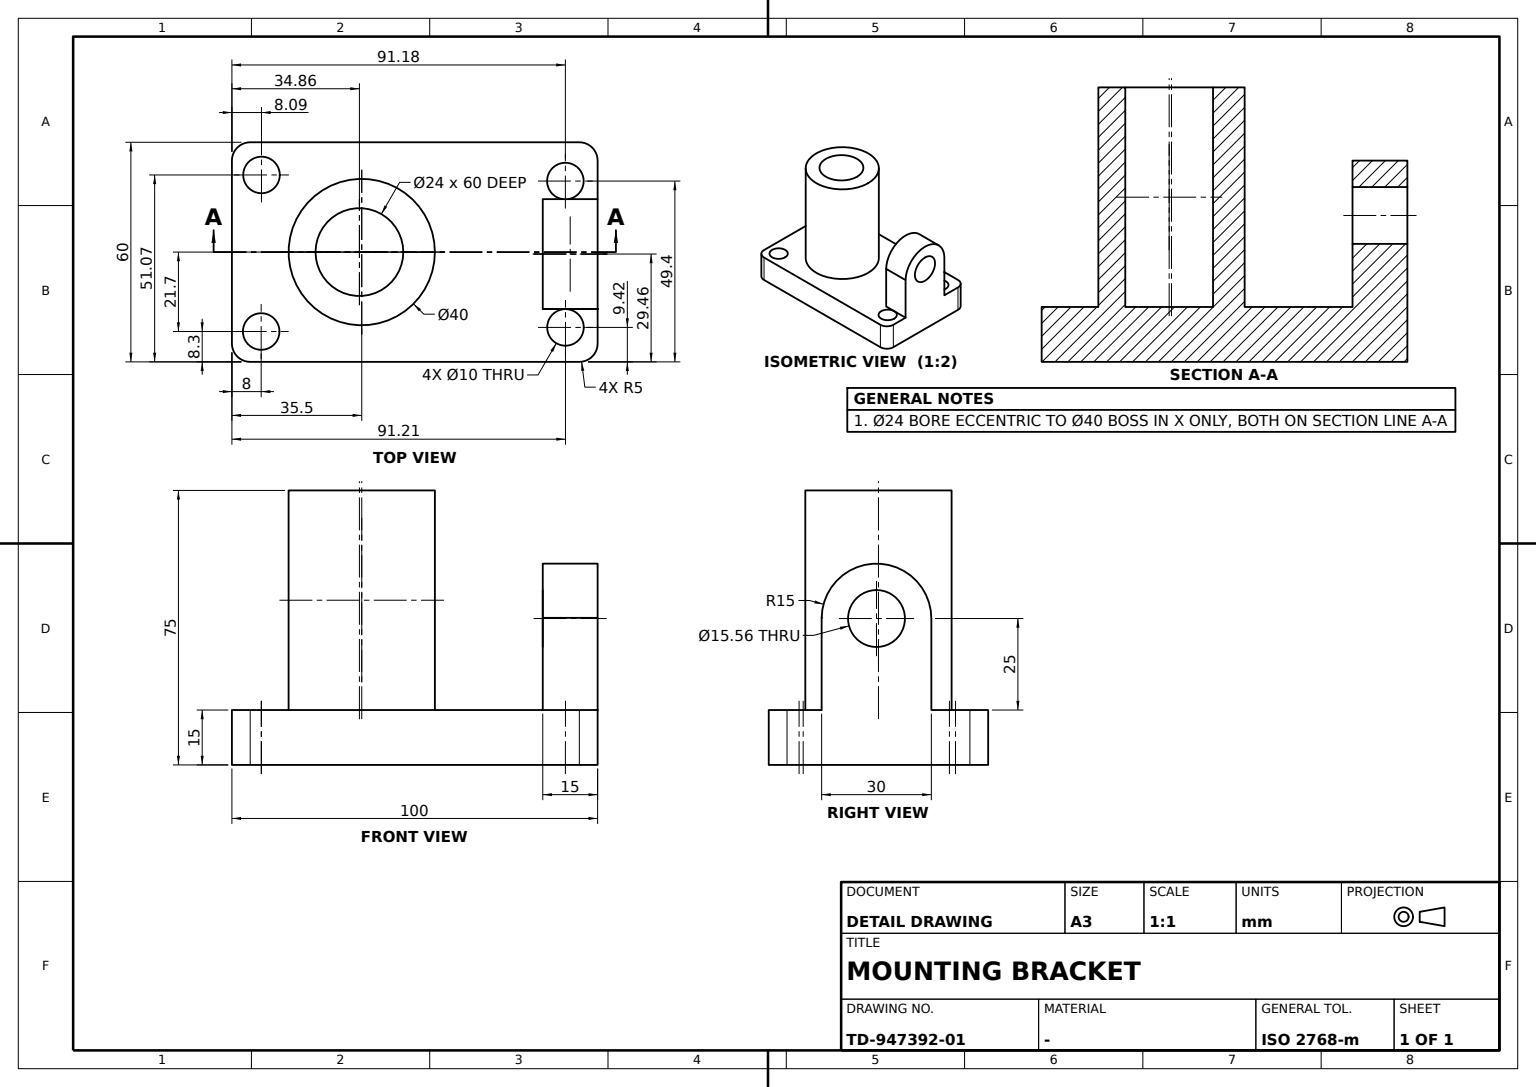
ISO-10303-21;
HEADER;
FILE_DESCRIPTION((''),'2;1');
FILE_NAME('','',(''),(''),'','','');
FILE_SCHEMA(('AUTOMOTIVE_DESIGN'));
ENDSEC;
DATA;
#1=APPLICATION_CONTEXT('');
#2=PRODUCT_CONTEXT('',#1,'mechanical');
#3=PRODUCT('','','',(#2));
#4=PRODUCT_DEFINITION_FORMATION('','',#3);
#5=PRODUCT_DEFINITION_CONTEXT('',#1,'design');
#6=PRODUCT_DEFINITION('','',#4,#5);
#7=PRODUCT_DEFINITION_SHAPE('','',#6);
#8=(LENGTH_UNIT()NAMED_UNIT(*)SI_UNIT(.MILLI.,.METRE.));
#9=(NAMED_UNIT(*)PLANE_ANGLE_UNIT()SI_UNIT($,.RADIAN.));
#10=(NAMED_UNIT(*)SI_UNIT($,.STERADIAN.)SOLID_ANGLE_UNIT());
#11=UNCERTAINTY_MEASURE_WITH_UNIT(LENGTH_MEASURE(0.005),#8,'distance_accuracy_value','');
#12=(GEOMETRIC_REPRESENTATION_CONTEXT(3)GLOBAL_UNCERTAINTY_ASSIGNED_CONTEXT((#11))GLOBAL_UNIT_ASSIGNED_CONTEXT((#8,#9,#10))REPRESENTATION_CONTEXT('',''));
#13=CARTESIAN_POINT('',(58.479646,14.464148,15.));
#14=VERTEX_POINT('',#13);
#15=CARTESIAN_POINT('',(60.042129,14.464148,15.));
#16=VERTEX_POINT('',#15);
#17=CARTESIAN_POINT('',(59.260888,19.402737,15.));
#18=DIRECTION('',(0.,0.,1.));
#19=DIRECTION('',(1.,0.,0.));
#20=AXIS2_PLACEMENT_3D('',#17,#18,#19);
#21=CIRCLE('',#20,5.);
#22=EDGE_CURVE('',#14,#16,#21,.T.);
#23=ORIENTED_EDGE('',*,*,#22,.F.);
#24=CARTESIAN_POINT('',(68.078188,14.464148,15.));
#25=DIRECTION('',(-1.,0.,0.));
#26=VECTOR('',#25,1000.);
#27=LINE('',#24,#26);
#28=EDGE_CURVE('',#16,#14,#27,.T.);
#29=ORIENTED_EDGE('',*,*,#28,.F.);
#30=EDGE_LOOP('',(#23,#29));
#31=FACE_BOUND('',#30,.T.);
#32=CARTESIAN_POINT('',(0.,0.,15.));
#33=AXIS2_PLACEMENT_3D('',#32,#18,#19);
#34=PLANE('',#33);
#35=ADVANCED_FACE('',(#31),#34,.F.);
#36=CARTESIAN_POINT('',(14.941721,0.,75.));
#37=VERTEX_POINT('',#36);
#38=CARTESIAN_POINT('',(2.941721,0.,75.));
#39=AXIS2_PLACEMENT_3D('',#38,#18,#19);
#40=CIRCLE('',#39,12.);
#41=EDGE_CURVE('',#37,#37,#40,.T.);
#42=ORIENTED_EDGE('',*,*,#41,.F.);
#43=EDGE_LOOP('',(#42));
#44=FACE_BOUND('',#43,.T.);
#45=CARTESIAN_POINT('',(23.581214,0.,75.));
#46=VERTEX_POINT('',#45);
#47=CARTESIAN_POINT('',(3.581214,0.,75.));
#48=AXIS2_PLACEMENT_3D('',#47,#18,#19);
#49=CIRCLE('',#48,20.);
#50=EDGE_CURVE('',#46,#46,#49,.T.);
#51=ORIENTED_EDGE('',*,*,#50,.T.);
#52=EDGE_LOOP('',(#51));
#53=FACE_BOUND('',#52,.T.);
#54=CARTESIAN_POINT('',(0.,0.,75.));
#55=AXIS2_PLACEMENT_3D('',#54,#18,#19);
#56=PLANE('',#55);
#57=ADVANCED_FACE('',(#44,#53),#56,.T.);
#58=CARTESIAN_POINT('',(68.078188,-15.536414,15.));
#59=VERTEX_POINT('',#58);
#60=CARTESIAN_POINT('',(53.078188,-15.536414,15.));
#61=VERTEX_POINT('',#60);
#62=CARTESIAN_POINT('',(0.,-15.536414,15.));
#63=LINE('',#62,#26);
#64=EDGE_CURVE('',#59,#61,#63,.T.);
#65=ORIENTED_EDGE('',*,*,#64,.F.);
#66=CARTESIAN_POINT('',(68.078188,-15.53529,40.183641));
#67=VERTEX_POINT('',#66);
#68=CARTESIAN_POINT('',(68.078188,-15.536414,0.));
#69=DIRECTION('',(0.,0.,-1.));
#70=VECTOR('',#69,1000.);
#71=LINE('',#68,#70);
#72=EDGE_CURVE('',#67,#59,#71,.T.);
#73=ORIENTED_EDGE('',*,*,#72,.F.);
#74=CARTESIAN_POINT('',(53.078188,-15.53529,40.18362));
#75=VERTEX_POINT('',#74);
#76=CARTESIAN_POINT('',(68.078188,-15.536414,40.18362));
#77=CARTESIAN_POINT('',(63.078188,-15.536414,40.18362));
#78=CARTESIAN_POINT('',(58.078188,-15.536414,40.18362));
#79=CARTESIAN_POINT('',(53.078188,-15.536414,40.18362));
#80=B_SPLINE_CURVE_WITH_KNOTS('',3,(#76,#77,#78,#79),.UNSPECIFIED.,.F.,.F.,(4,4),(0.,1.),.UNSPECIFIED.);
#81=EDGE_CURVE('',#67,#75,#80,.T.);
#82=ORIENTED_EDGE('',*,*,#81,.T.);
#83=LINE('',#79,#70);
#84=EDGE_CURVE('',#75,#61,#83,.T.);
#85=ORIENTED_EDGE('',*,*,#84,.T.);
#86=EDGE_LOOP('',(#65,#73,#82,#85));
#87=FACE_BOUND('',#86,.T.);
#88=DIRECTION('',(0.,1.,0.));
#89=AXIS2_PLACEMENT_3D('',#76,#88,#69);
#90=PLANE('',#89);
#91=ADVANCED_FACE('',(#87),#90,.F.);
#92=CARTESIAN_POINT('',(-26.921812,-30.,0.));
#93=VERTEX_POINT('',#92);
#94=CARTESIAN_POINT('',(-26.921812,-30.,15.));
#95=VERTEX_POINT('',#94);
#96=CARTESIAN_POINT('',(-26.921812,-30.,7.5));
#97=VECTOR('',#18,1000.);
#98=LINE('',#96,#97);
#99=EDGE_CURVE('',#93,#95,#98,.T.);
#100=ORIENTED_EDGE('',*,*,#99,.F.);
#101=CARTESIAN_POINT('',(63.078188,-30.,0.));
#102=VERTEX_POINT('',#101);
#103=CARTESIAN_POINT('',(0.,-30.,0.));
#104=LINE('',#103,#26);
#105=EDGE_CURVE('',#102,#93,#104,.T.);
#106=ORIENTED_EDGE('',*,*,#105,.F.);
#107=CARTESIAN_POINT('',(63.078188,-30.,15.));
#108=VERTEX_POINT('',#107);
#109=CARTESIAN_POINT('',(63.078188,-30.,7.5));
#110=LINE('',#109,#97);
#111=EDGE_CURVE('',#102,#108,#110,.T.);
#112=ORIENTED_EDGE('',*,*,#111,.T.);
#113=CARTESIAN_POINT('',(0.,-30.,15.));
#114=LINE('',#113,#26);
#115=EDGE_CURVE('',#108,#95,#114,.T.);
#116=ORIENTED_EDGE('',*,*,#115,.T.);
#117=EDGE_LOOP('',(#100,#106,#112,#116));
#118=FACE_BOUND('',#117,.T.);
#119=AXIS2_PLACEMENT_3D('',#101,#88,#25);
#120=PLANE('',#119);
#121=ADVANCED_FACE('',(#118),#120,.F.);
#122=CARTESIAN_POINT('',(-18.830684,21.069996,0.));
#123=VERTEX_POINT('',#122);
#124=CARTESIAN_POINT('',(-23.830684,21.069996,0.));
#125=AXIS2_PLACEMENT_3D('',#124,#18,#19);
#126=CIRCLE('',#125,5.);
#127=EDGE_CURVE('',#123,#123,#126,.T.);
#128=ORIENTED_EDGE('',*,*,#127,.F.);
#129=EDGE_LOOP('',(#128));
#130=FACE_BOUND('',#129,.T.);
#131=CARTESIAN_POINT('',(-18.830684,21.069996,15.));
#132=VERTEX_POINT('',#131);
#133=CARTESIAN_POINT('',(-23.830684,21.069996,15.));
#134=AXIS2_PLACEMENT_3D('',#133,#18,#19);
#135=CIRCLE('',#134,5.);
#136=EDGE_CURVE('',#132,#132,#135,.T.);
#137=ORIENTED_EDGE('',*,*,#136,.T.);
#138=EDGE_LOOP('',(#137));
#139=FACE_BOUND('',#138,.T.);
#140=CARTESIAN_POINT('',(-23.830684,21.069996,7.5));
#141=AXIS2_PLACEMENT_3D('',#140,#18,#19);
#142=CYLINDRICAL_SURFACE('',#141,5.);
#143=ADVANCED_FACE('',(#130,#139),#142,.F.);
#144=CARTESIAN_POINT('',(-18.919036,-21.704368,15.));
#145=VERTEX_POINT('',#144);
#146=CARTESIAN_POINT('',(-23.919036,-21.704368,15.));
#147=AXIS2_PLACEMENT_3D('',#146,#18,#19);
#148=CIRCLE('',#147,5.);
#149=EDGE_CURVE('',#145,#145,#148,.T.);
#150=ORIENTED_EDGE('',*,*,#149,.F.);
#151=EDGE_LOOP('',(#150));
#152=FACE_BOUND('',#151,.T.);
#153=CARTESIAN_POINT('',(23.581214,0.,15.));
#154=VERTEX_POINT('',#153);
#155=CARTESIAN_POINT('',(3.581214,0.,15.));
#156=AXIS2_PLACEMENT_3D('',#155,#18,#19);
#157=CIRCLE('',#156,20.);
#158=EDGE_CURVE('',#154,#154,#157,.T.);
#159=ORIENTED_EDGE('',*,*,#158,.F.);
#160=EDGE_LOOP('',(#159));
#161=FACE_BOUND('',#160,.T.);
#162=CARTESIAN_POINT('',(64.287583,-20.583682,15.));
#163=VERTEX_POINT('',#162);
#164=CARTESIAN_POINT('',(59.287583,-20.583682,15.));
#165=AXIS2_PLACEMENT_3D('',#164,#18,#19);
#166=CIRCLE('',#165,5.);
#167=EDGE_CURVE('',#163,#163,#166,.T.);
#168=ORIENTED_EDGE('',*,*,#167,.F.);
#169=EDGE_LOOP('',(#168));
#170=FACE_BOUND('',#169,.T.);
#171=ORIENTED_EDGE('',*,*,#136,.F.);
#172=EDGE_LOOP('',(#171));
#173=FACE_BOUND('',#172,.T.);
#174=CARTESIAN_POINT('',(68.078188,-25.,15.));
#175=VERTEX_POINT('',#174);
#176=CARTESIAN_POINT('',(68.078188,0.,15.));
#177=DIRECTION('',(0.,-1.,0.));
#178=VECTOR('',#177,1000.);
#179=LINE('',#176,#178);
#180=EDGE_CURVE('',#59,#175,#179,.T.);
#181=ORIENTED_EDGE('',*,*,#180,.F.);
#182=ORIENTED_EDGE('',*,*,#64,.T.);
#183=CARTESIAN_POINT('',(53.078188,14.464148,15.));
#184=VERTEX_POINT('',#183);
#185=CARTESIAN_POINT('',(53.078188,0.,15.));
#186=VECTOR('',#88,1000.);
#187=LINE('',#185,#186);
#188=EDGE_CURVE('',#61,#184,#187,.T.);
#189=ORIENTED_EDGE('',*,*,#188,.T.);
#190=EDGE_CURVE('',#14,#184,#27,.T.);
#191=ORIENTED_EDGE('',*,*,#190,.F.);
#192=EDGE_CURVE('',#16,#14,#21,.T.);
#193=ORIENTED_EDGE('',*,*,#192,.F.);
#194=VERTEX_POINT('',#24);
#195=EDGE_CURVE('',#194,#16,#27,.T.);
#196=ORIENTED_EDGE('',*,*,#195,.F.);
#197=CARTESIAN_POINT('',(68.078188,25.,15.));
#198=VERTEX_POINT('',#197);
#199=EDGE_CURVE('',#198,#194,#179,.T.);
#200=ORIENTED_EDGE('',*,*,#199,.F.);
#201=CARTESIAN_POINT('',(63.078188,30.,15.));
#202=VERTEX_POINT('',#201);
#203=CARTESIAN_POINT('',(63.078188,25.,15.));
#204=AXIS2_PLACEMENT_3D('',#203,#18,#19);
#205=CIRCLE('',#204,5.);
#206=EDGE_CURVE('',#198,#202,#205,.T.);
#207=ORIENTED_EDGE('',*,*,#206,.T.);
#208=CARTESIAN_POINT('',(-26.921812,30.,15.));
#209=VERTEX_POINT('',#208);
#210=CARTESIAN_POINT('',(0.,30.,15.));
#211=VECTOR('',#19,1000.);
#212=LINE('',#210,#211);
#213=EDGE_CURVE('',#209,#202,#212,.T.);
#214=ORIENTED_EDGE('',*,*,#213,.F.);
#215=CARTESIAN_POINT('',(-31.921812,25.,15.));
#216=VERTEX_POINT('',#215);
#217=CARTESIAN_POINT('',(-26.921812,25.,15.));
#218=AXIS2_PLACEMENT_3D('',#217,#18,#19);
#219=CIRCLE('',#218,5.);
#220=EDGE_CURVE('',#209,#216,#219,.T.);
#221=ORIENTED_EDGE('',*,*,#220,.T.);
#222=CARTESIAN_POINT('',(-31.921812,-25.,15.));
#223=VERTEX_POINT('',#222);
#224=CARTESIAN_POINT('',(-31.921812,0.,15.));
#225=LINE('',#224,#186);
#226=EDGE_CURVE('',#223,#216,#225,.T.);
#227=ORIENTED_EDGE('',*,*,#226,.F.);
#228=CARTESIAN_POINT('',(-26.921812,-25.,15.));
#229=AXIS2_PLACEMENT_3D('',#228,#18,#19);
#230=CIRCLE('',#229,5.);
#231=EDGE_CURVE('',#223,#95,#230,.T.);
#232=ORIENTED_EDGE('',*,*,#231,.T.);
#233=ORIENTED_EDGE('',*,*,#115,.F.);
#234=CARTESIAN_POINT('',(63.078188,-25.,15.));
#235=AXIS2_PLACEMENT_3D('',#234,#18,#19);
#236=CIRCLE('',#235,5.);
#237=EDGE_CURVE('',#108,#175,#236,.T.);
#238=ORIENTED_EDGE('',*,*,#237,.T.);
#239=EDGE_LOOP('',(#181,#182,#189,#191,#193,#196,#200,#207,#214,#221,#227,#232,#233,#238));
#240=FACE_BOUND('',#239,.T.);
#241=ADVANCED_FACE('',(#152,#161,#170,#173,#240),#34,.T.);
#242=CARTESIAN_POINT('',(68.078188,-0.536133,47.780245));
#243=VERTEX_POINT('',#242);
#244=CARTESIAN_POINT('',(68.078188,-0.536133,40.));
#245=AXIS2_PLACEMENT_3D('',#244,#25,#18);
#246=CIRCLE('',#245,7.780245);
#247=EDGE_CURVE('',#243,#243,#246,.F.);
#248=ORIENTED_EDGE('',*,*,#247,.F.);
#249=EDGE_LOOP('',(#248));
#250=FACE_BOUND('',#249,.T.);
#251=ORIENTED_EDGE('',*,*,#72,.T.);
#252=ORIENTED_EDGE('',*,*,#180,.T.);
#253=CARTESIAN_POINT('',(68.078188,-25.,0.));
#254=VERTEX_POINT('',#253);
#255=CARTESIAN_POINT('',(68.078188,-25.,7.5));
#256=LINE('',#255,#97);
#257=EDGE_CURVE('',#254,#175,#256,.T.);
#258=ORIENTED_EDGE('',*,*,#257,.F.);
#259=CARTESIAN_POINT('',(68.078188,25.,0.));
#260=VERTEX_POINT('',#259);
#261=CARTESIAN_POINT('',(68.078188,0.,0.));
#262=LINE('',#261,#178);
#263=EDGE_CURVE('',#260,#254,#262,.T.);
#264=ORIENTED_EDGE('',*,*,#263,.F.);
#265=CARTESIAN_POINT('',(68.078188,25.,7.5));
#266=LINE('',#265,#97);
#267=EDGE_CURVE('',#260,#198,#266,.T.);
#268=ORIENTED_EDGE('',*,*,#267,.T.);
#269=ORIENTED_EDGE('',*,*,#199,.T.);
#270=CARTESIAN_POINT('',(68.078188,14.464148,40.));
#271=VERTEX_POINT('',#270);
#272=CARTESIAN_POINT('',(68.078188,14.464148,0.));
#273=LINE('',#272,#97);
#274=EDGE_CURVE('',#194,#271,#273,.T.);
#275=ORIENTED_EDGE('',*,*,#274,.T.);
#276=CIRCLE('',#245,15.000281);
#277=EDGE_CURVE('',#271,#67,#276,.F.);
#278=ORIENTED_EDGE('',*,*,#277,.T.);
#279=EDGE_LOOP('',(#251,#252,#258,#264,#268,#269,#275,#278));
#280=FACE_BOUND('',#279,.T.);
#281=AXIS2_PLACEMENT_3D('',#259,#25,#177);
#282=PLANE('',#281);
#283=ADVANCED_FACE('',(#250,#280),#282,.F.);
#284=CARTESIAN_POINT('',(53.078188,-0.536133,32.219755));
#285=VERTEX_POINT('',#284);
#286=CARTESIAN_POINT('',(53.078188,-0.536133,40.));
#287=AXIS2_PLACEMENT_3D('',#286,#19,#69);
#288=CIRCLE('',#287,7.780245);
#289=EDGE_CURVE('',#285,#285,#288,.T.);
#290=ORIENTED_EDGE('',*,*,#289,.F.);
#291=EDGE_LOOP('',(#290));
#292=FACE_BOUND('',#291,.T.);
#293=ORIENTED_EDGE('',*,*,#247,.T.);
#294=EDGE_LOOP('',(#293));
#295=FACE_BOUND('',#294,.T.);
#296=CARTESIAN_POINT('',(60.578188,-0.536133,40.));
#297=AXIS2_PLACEMENT_3D('',#296,#19,#88);
#298=CYLINDRICAL_SURFACE('',#297,7.780245);
#299=ADVANCED_FACE('',(#292,#295),#298,.F.);
#300=CARTESIAN_POINT('',(64.287583,-20.583682,0.));
#301=VERTEX_POINT('',#300);
#302=CARTESIAN_POINT('',(59.287583,-20.583682,0.));
#303=AXIS2_PLACEMENT_3D('',#302,#18,#19);
#304=CIRCLE('',#303,5.);
#305=EDGE_CURVE('',#301,#301,#304,.T.);
#306=ORIENTED_EDGE('',*,*,#305,.F.);
#307=EDGE_LOOP('',(#306));
#308=FACE_BOUND('',#307,.T.);
#309=ORIENTED_EDGE('',*,*,#167,.T.);
#310=EDGE_LOOP('',(#309));
#311=FACE_BOUND('',#310,.T.);
#312=CARTESIAN_POINT('',(59.287583,-20.583682,7.5));
#313=AXIS2_PLACEMENT_3D('',#312,#18,#19);
#314=CYLINDRICAL_SURFACE('',#313,5.);
#315=ADVANCED_FACE('',(#308,#311),#314,.F.);
#316=CARTESIAN_POINT('',(14.941721,0.,15.));
#317=VERTEX_POINT('',#316);
#318=CARTESIAN_POINT('',(2.941721,0.,15.));
#319=AXIS2_PLACEMENT_3D('',#318,#18,#19);
#320=CIRCLE('',#319,12.);
#321=EDGE_CURVE('',#317,#317,#320,.T.);
#322=ORIENTED_EDGE('',*,*,#321,.T.);
#323=EDGE_LOOP('',(#322));
#324=FACE_BOUND('',#323,.T.);
#325=ADVANCED_FACE('',(#324),#34,.T.);
#326=CARTESIAN_POINT('',(-18.919036,-21.704368,0.));
#327=VERTEX_POINT('',#326);
#328=CARTESIAN_POINT('',(-23.919036,-21.704368,0.));
#329=AXIS2_PLACEMENT_3D('',#328,#18,#19);
#330=CIRCLE('',#329,5.);
#331=EDGE_CURVE('',#327,#327,#330,.T.);
#332=ORIENTED_EDGE('',*,*,#331,.F.);
#333=EDGE_LOOP('',(#332));
#334=FACE_BOUND('',#333,.T.);
#335=ORIENTED_EDGE('',*,*,#149,.T.);
#336=EDGE_LOOP('',(#335));
#337=FACE_BOUND('',#336,.T.);
#338=CARTESIAN_POINT('',(-23.919036,-21.704368,7.5));
#339=AXIS2_PLACEMENT_3D('',#338,#18,#19);
#340=CYLINDRICAL_SURFACE('',#339,5.);
#341=ADVANCED_FACE('',(#334,#337),#340,.F.);
#342=CARTESIAN_POINT('',(53.078188,14.464148,40.));
#343=VERTEX_POINT('',#342);
#344=LINE('',#183,#97);
#345=EDGE_CURVE('',#184,#343,#344,.T.);
#346=ORIENTED_EDGE('',*,*,#345,.F.);
#347=ORIENTED_EDGE('',*,*,#188,.F.);
#348=ORIENTED_EDGE('',*,*,#84,.F.);
#349=CIRCLE('',#287,15.000281);
#350=EDGE_CURVE('',#343,#75,#349,.T.);
#351=ORIENTED_EDGE('',*,*,#350,.F.);
#352=EDGE_LOOP('',(#346,#347,#348,#351));
#353=FACE_BOUND('',#352,.T.);
#354=ORIENTED_EDGE('',*,*,#289,.T.);
#355=EDGE_LOOP('',(#354));
#356=FACE_BOUND('',#355,.T.);
#357=CARTESIAN_POINT('',(53.078188,0.,0.));
#358=AXIS2_PLACEMENT_3D('',#357,#19,#88);
#359=PLANE('',#358);
#360=ADVANCED_FACE('',(#353,#356),#359,.F.);
#361=ORIENTED_EDGE('',*,*,#213,.T.);
#362=CARTESIAN_POINT('',(63.078188,30.,0.));
#363=VERTEX_POINT('',#362);
#364=CARTESIAN_POINT('',(63.078188,30.,7.5));
#365=LINE('',#364,#97);
#366=EDGE_CURVE('',#363,#202,#365,.T.);
#367=ORIENTED_EDGE('',*,*,#366,.F.);
#368=CARTESIAN_POINT('',(-26.921812,30.,0.));
#369=VERTEX_POINT('',#368);
#370=CARTESIAN_POINT('',(0.,30.,0.));
#371=LINE('',#370,#211);
#372=EDGE_CURVE('',#369,#363,#371,.T.);
#373=ORIENTED_EDGE('',*,*,#372,.F.);
#374=CARTESIAN_POINT('',(-26.921812,30.,7.5));
#375=LINE('',#374,#97);
#376=EDGE_CURVE('',#369,#209,#375,.T.);
#377=ORIENTED_EDGE('',*,*,#376,.T.);
#378=EDGE_LOOP('',(#361,#367,#373,#377));
#379=FACE_BOUND('',#378,.T.);
#380=AXIS2_PLACEMENT_3D('',#368,#177,#19);
#381=PLANE('',#380);
#382=ADVANCED_FACE('',(#379),#381,.F.);
#383=ORIENTED_EDGE('',*,*,#206,.F.);
#384=ORIENTED_EDGE('',*,*,#267,.F.);
#385=CARTESIAN_POINT('',(63.078188,25.,0.));
#386=AXIS2_PLACEMENT_3D('',#385,#18,#19);
#387=CIRCLE('',#386,5.);
#388=EDGE_CURVE('',#260,#363,#387,.T.);
#389=ORIENTED_EDGE('',*,*,#388,.T.);
#390=ORIENTED_EDGE('',*,*,#366,.T.);
#391=EDGE_LOOP('',(#383,#384,#389,#390));
#392=FACE_BOUND('',#391,.T.);
#393=CARTESIAN_POINT('',(63.078188,25.,7.5));
#394=AXIS2_PLACEMENT_3D('',#393,#18,#19);
#395=CYLINDRICAL_SURFACE('',#394,5.);
#396=ADVANCED_FACE('',(#392),#395,.T.);
#397=ORIENTED_EDGE('',*,*,#274,.F.);
#398=ORIENTED_EDGE('',*,*,#195,.T.);
#399=ORIENTED_EDGE('',*,*,#28,.T.);
#400=ORIENTED_EDGE('',*,*,#190,.T.);
#401=ORIENTED_EDGE('',*,*,#345,.T.);
#402=CARTESIAN_POINT('',(60.578188,14.464148,40.));
#403=LINE('',#402,#211);
#404=EDGE_CURVE('',#271,#343,#403,.F.);
#405=ORIENTED_EDGE('',*,*,#404,.F.);
#406=EDGE_LOOP('',(#397,#398,#399,#400,#401,#405));
#407=FACE_BOUND('',#406,.T.);
#408=AXIS2_PLACEMENT_3D('',#24,#177,#18);
#409=PLANE('',#408);
#410=ADVANCED_FACE('',(#407),#409,.F.);
#411=ORIENTED_EDGE('',*,*,#388,.F.);
#412=ORIENTED_EDGE('',*,*,#263,.T.);
#413=CARTESIAN_POINT('',(63.078188,-25.,0.));
#414=AXIS2_PLACEMENT_3D('',#413,#18,#19);
#415=CIRCLE('',#414,5.);
#416=EDGE_CURVE('',#102,#254,#415,.T.);
#417=ORIENTED_EDGE('',*,*,#416,.F.);
#418=ORIENTED_EDGE('',*,*,#105,.T.);
#419=CARTESIAN_POINT('',(-31.921812,-25.,0.));
#420=VERTEX_POINT('',#419);
#421=CARTESIAN_POINT('',(-26.921812,-25.,0.));
#422=AXIS2_PLACEMENT_3D('',#421,#18,#19);
#423=CIRCLE('',#422,5.);
#424=EDGE_CURVE('',#420,#93,#423,.T.);
#425=ORIENTED_EDGE('',*,*,#424,.F.);
#426=CARTESIAN_POINT('',(-31.921812,25.,0.));
#427=VERTEX_POINT('',#426);
#428=CARTESIAN_POINT('',(-31.921812,0.,0.));
#429=LINE('',#428,#186);
#430=EDGE_CURVE('',#420,#427,#429,.T.);
#431=ORIENTED_EDGE('',*,*,#430,.T.);
#432=CARTESIAN_POINT('',(-26.921812,25.,0.));
#433=AXIS2_PLACEMENT_3D('',#432,#18,#19);
#434=CIRCLE('',#433,5.);
#435=EDGE_CURVE('',#369,#427,#434,.T.);
#436=ORIENTED_EDGE('',*,*,#435,.F.);
#437=ORIENTED_EDGE('',*,*,#372,.T.);
#438=EDGE_LOOP('',(#411,#412,#417,#418,#425,#431,#436,#437));
#439=FACE_BOUND('',#438,.T.);
#440=ORIENTED_EDGE('',*,*,#305,.T.);
#441=EDGE_LOOP('',(#440));
#442=FACE_BOUND('',#441,.T.);
#443=ORIENTED_EDGE('',*,*,#127,.T.);
#444=EDGE_LOOP('',(#443));
#445=FACE_BOUND('',#444,.T.);
#446=ORIENTED_EDGE('',*,*,#331,.T.);
#447=EDGE_LOOP('',(#446));
#448=FACE_BOUND('',#447,.T.);
#449=CARTESIAN_POINT('',(64.260888,19.402737,0.));
#450=VERTEX_POINT('',#449);
#451=CARTESIAN_POINT('',(59.260888,19.402737,0.));
#452=AXIS2_PLACEMENT_3D('',#451,#18,#19);
#453=CIRCLE('',#452,5.);
#454=EDGE_CURVE('',#450,#450,#453,.T.);
#455=ORIENTED_EDGE('',*,*,#454,.T.);
#456=EDGE_LOOP('',(#455));
#457=FACE_BOUND('',#456,.T.);
#458=CARTESIAN_POINT('',(0.,0.,0.));
#459=AXIS2_PLACEMENT_3D('',#458,#18,#19);
#460=PLANE('',#459);
#461=ADVANCED_FACE('',(#439,#442,#445,#448,#457),#460,.F.);
#462=ORIENTED_EDGE('',*,*,#231,.F.);
#463=CARTESIAN_POINT('',(-31.921812,-25.,7.5));
#464=LINE('',#463,#97);
#465=EDGE_CURVE('',#420,#223,#464,.T.);
#466=ORIENTED_EDGE('',*,*,#465,.F.);
#467=ORIENTED_EDGE('',*,*,#424,.T.);
#468=ORIENTED_EDGE('',*,*,#99,.T.);
#469=EDGE_LOOP('',(#462,#466,#467,#468));
#470=FACE_BOUND('',#469,.T.);
#471=CARTESIAN_POINT('',(-26.921812,-25.,7.5));
#472=AXIS2_PLACEMENT_3D('',#471,#18,#19);
#473=CYLINDRICAL_SURFACE('',#472,5.);
#474=ADVANCED_FACE('',(#470),#473,.T.);
#475=ORIENTED_EDGE('',*,*,#321,.F.);
#476=EDGE_LOOP('',(#475));
#477=FACE_BOUND('',#476,.T.);
#478=ORIENTED_EDGE('',*,*,#41,.T.);
#479=EDGE_LOOP('',(#478));
#480=FACE_BOUND('',#479,.T.);
#481=CARTESIAN_POINT('',(2.941721,0.,45.));
#482=AXIS2_PLACEMENT_3D('',#481,#18,#19);
#483=CYLINDRICAL_SURFACE('',#482,12.);
#484=ADVANCED_FACE('',(#477,#480),#483,.F.);
#485=ORIENTED_EDGE('',*,*,#257,.T.);
#486=ORIENTED_EDGE('',*,*,#237,.F.);
#487=ORIENTED_EDGE('',*,*,#111,.F.);
#488=ORIENTED_EDGE('',*,*,#416,.T.);
#489=EDGE_LOOP('',(#485,#486,#487,#488));
#490=FACE_BOUND('',#489,.T.);
#491=CARTESIAN_POINT('',(63.078188,-25.,7.5));
#492=AXIS2_PLACEMENT_3D('',#491,#18,#19);
#493=CYLINDRICAL_SURFACE('',#492,5.);
#494=ADVANCED_FACE('',(#490),#493,.T.);
#495=ORIENTED_EDGE('',*,*,#465,.T.);
#496=ORIENTED_EDGE('',*,*,#226,.T.);
#497=CARTESIAN_POINT('',(-31.921812,25.,7.5));
#498=LINE('',#497,#97);
#499=EDGE_CURVE('',#427,#216,#498,.T.);
#500=ORIENTED_EDGE('',*,*,#499,.F.);
#501=ORIENTED_EDGE('',*,*,#430,.F.);
#502=EDGE_LOOP('',(#495,#496,#500,#501));
#503=FACE_BOUND('',#502,.T.);
#504=AXIS2_PLACEMENT_3D('',#419,#19,#88);
#505=PLANE('',#504);
#506=ADVANCED_FACE('',(#503),#505,.F.);
#507=ORIENTED_EDGE('',*,*,#454,.F.);
#508=EDGE_LOOP('',(#507));
#509=FACE_BOUND('',#508,.T.);
#510=ORIENTED_EDGE('',*,*,#22,.T.);
#511=ORIENTED_EDGE('',*,*,#192,.T.);
#512=EDGE_LOOP('',(#510,#511));
#513=FACE_BOUND('',#512,.T.);
#514=CARTESIAN_POINT('',(59.260888,19.402737,7.5));
#515=AXIS2_PLACEMENT_3D('',#514,#18,#19);
#516=CYLINDRICAL_SURFACE('',#515,5.);
#517=ADVANCED_FACE('',(#509,#513),#516,.F.);
#518=ORIENTED_EDGE('',*,*,#404,.T.);
#519=ORIENTED_EDGE('',*,*,#350,.T.);
#520=ORIENTED_EDGE('',*,*,#81,.F.);
#521=ORIENTED_EDGE('',*,*,#277,.F.);
#522=EDGE_LOOP('',(#518,#519,#520,#521));
#523=FACE_BOUND('',#522,.T.);
#524=CYLINDRICAL_SURFACE('',#297,15.000281);
#525=ADVANCED_FACE('',(#523),#524,.T.);
#526=ORIENTED_EDGE('',*,*,#158,.T.);
#527=EDGE_LOOP('',(#526));
#528=FACE_BOUND('',#527,.T.);
#529=ORIENTED_EDGE('',*,*,#50,.F.);
#530=EDGE_LOOP('',(#529));
#531=FACE_BOUND('',#530,.T.);
#532=CARTESIAN_POINT('',(3.581214,0.,45.));
#533=AXIS2_PLACEMENT_3D('',#532,#18,#19);
#534=CYLINDRICAL_SURFACE('',#533,20.);
#535=ADVANCED_FACE('',(#528,#531),#534,.T.);
#536=ORIENTED_EDGE('',*,*,#376,.F.);
#537=ORIENTED_EDGE('',*,*,#435,.T.);
#538=ORIENTED_EDGE('',*,*,#499,.T.);
#539=ORIENTED_EDGE('',*,*,#220,.F.);
#540=EDGE_LOOP('',(#536,#537,#538,#539));
#541=FACE_BOUND('',#540,.T.);
#542=CARTESIAN_POINT('',(-26.921812,25.,7.5));
#543=AXIS2_PLACEMENT_3D('',#542,#18,#19);
#544=CYLINDRICAL_SURFACE('',#543,5.);
#545=ADVANCED_FACE('',(#541),#544,.T.);
#546=CLOSED_SHELL('',(#35,#57,#91,#121,#143,#241,#283,#299,#315,#325,#341,#360,#382,#396,#410,#461,#474,#484,#494,#506,#517,#525,#535,#545));
#547=MANIFOLD_SOLID_BREP('',#546);
#548=ADVANCED_BREP_SHAPE_REPRESENTATION('',(#547),#12);
#549=SHAPE_DEFINITION_REPRESENTATION(#7,#548);
ENDSEC;
END-ISO-10303-21;
